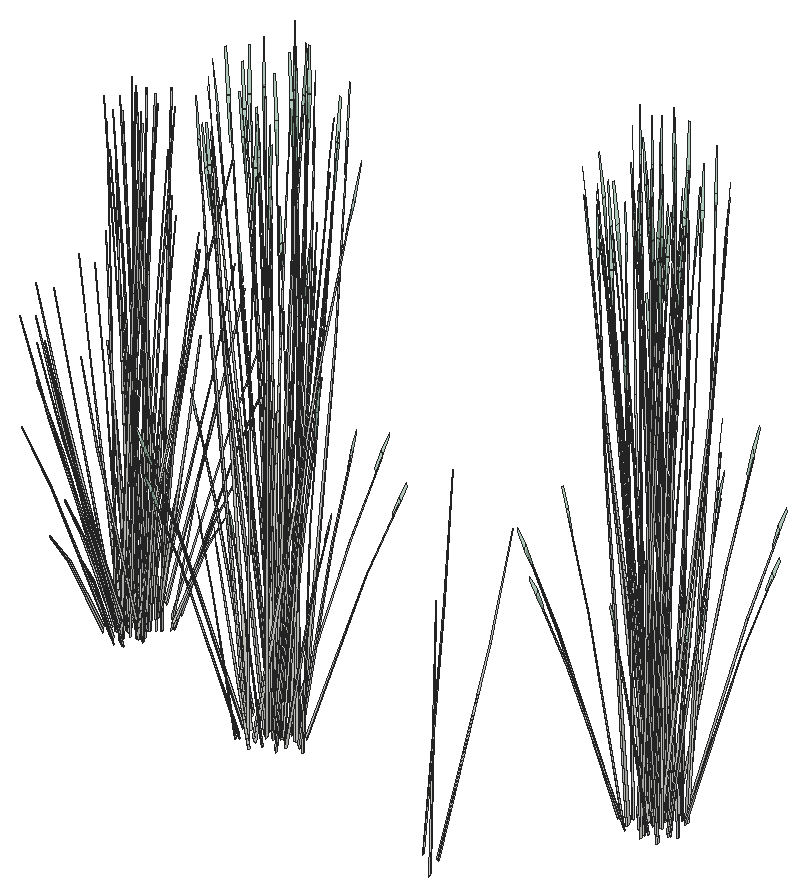
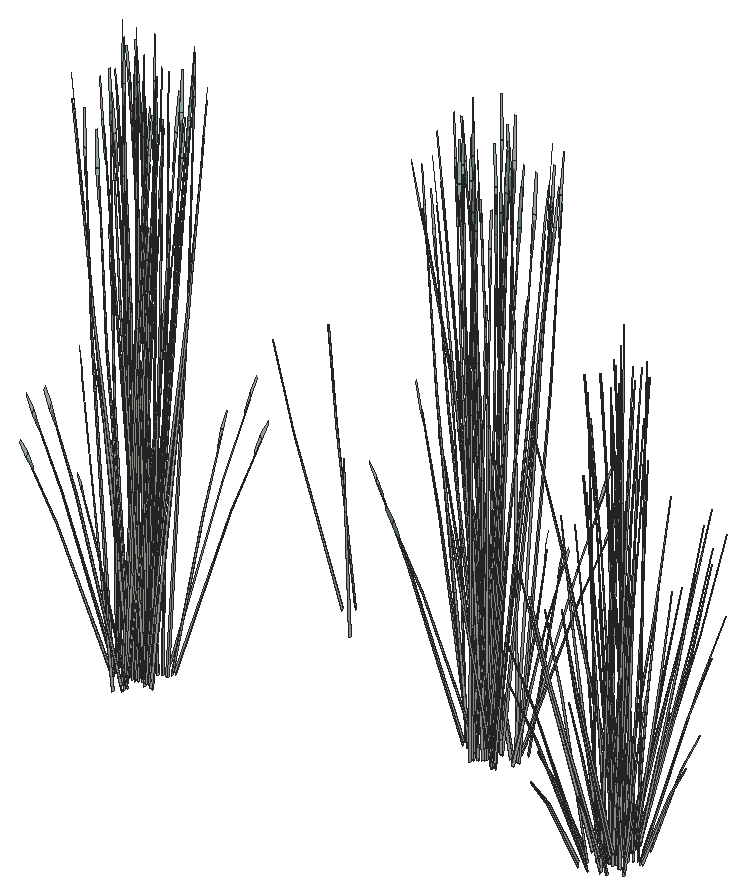
# SketchUp Ruby script. Lengths in inches.
U = 1.inch
M = Sketchup.active_model
def pt(a) = Geom::Point3d.new(a.map { |v| v * U })
def face(e, loops, mat)
  f = e.add_face(loops[0].map { |a| pt(a) })
  loops[1..].each { |l| e.add_face(l.map { |a| pt(a) }).erase! }
  f.material = f.back_material = mat if mat
  f
end
# faces: each face lists its corners as indices into pts; further lists are holes
def faces(e, pts, list, mat = nil) = list.each { |f| face(e, (f[0].is_a?(Array) ? f : [f]).map { |l| l.map { |i| pts[i] } }, mat) }
# xy, xz, yz: faces in a plane at the given z, y or x. An outline is a flat list of corners, or four numbers for a rectangle; further outlines are holes
def ring(l) = l.size == 4 ? [[l[0], l[1]], [l[2], l[1]], [l[2], l[3]], [l[0], l[3]]] : l.each_slice(2).to_a
def flat(e, list, mat, &to3) = list.each { |f| face(e, (f[0].is_a?(Array) ? f : [f]).map { |l| ring(l).map { |u, v| to3.(u, v) } }, mat) }
def xy(e, z, list, mat = nil) = flat(e, list, mat) { |x, y| [x, y, z] }
def xz(e, y, list, mat = nil) = flat(e, list, mat) { |x, z| [x, y, z] }
def yz(e, x, list, mat = nil) = flat(e, list, mat) { |y, z| [x, y, z] }
def lines(e, pts, list) = list.each { |a, b| e.add_line(pt(pts[a]), pt(pts[b])) }
# prism: a flat outline (further loops are holes) pulled along v
def prism(e, loops, v, mat = nil)
  f = face(e, loops, mat); d = Geom::Vector3d.new(v.map { |x| x * U })
  f.pushpull(f.normal.samedirection?(d) ? d.length : -d.length)
end
def box(e, o, s, mat = nil) = prism(e, [[o, [o[0] + s[0], o[1], o[2]], [o[0] + s[0], o[1] + s[1], o[2]], [o[0], o[1] + s[1], o[2]]]], [0, 0, s[2]], mat)
def at(x, y, z, deg = 0) = Geom::Transformation.translation(pt([x, y, z])) * Geom::Transformation.rotation(ORIGIN, Z_AXIS, deg.degrees)
def axes(o, x, y, z) = Geom::Transformation.new([*x, 0, *y, 0, *z, 0, *pt(o).to_a, 1])
def part(name) = M.definitions.add(name)
# library, detail: a bought-in or finely detailed component or shape, given as its bounding box
def library(name, o, s) = part(name).tap { |d| box(d.entities, o, s) }
def detail(e, o, s) = box(e.add_group.entities, o, s)
def put(e, d, t, mat = nil) = e.add_instance(d, t).tap { |i| i.material = mat if mat }
def group(e, t, mat = nil) = e.add_group.tap { |g| g.transformation = t; g.material = mat if mat }.entities
root = M.entities
M.materials.add("LightPink_Translucent").color = [175, 214, 192]
M.materials["LightPink_Translucent"].alpha = 0.75
c1 = part("blade")
p = [[2.15,0.21,22],[0,0.17,0],[0.09,0.45,0],[2.18,0.31,22],[2.29,0.31,22],[0.38,0.45,0],
  [2.48,0.24,33],[2.49,0.24,33],[2.48,0.22,33]]
faces(c1.entities,p,[[0,1,2,3],[4,5,2,3],[6,3,4,7],[8,0,3,6]])
c2 = part("blade with seeds\#1")
put(c2.entities,c1,at(0,0,0))
c3 = part("seeds")
p = [[0.3,-0.1,1.38],[-0.01,-0.03,1.59],[-0.01,-0.03,0.03],[0.14,-0.07,-0.07],[0.29,-0.03,3],[0.15,0.01,3.11]]
faces(c3.entities,p,[[0,1,2,3],[1,0,4,5]],"LightPink_Translucent")
c4 = part("blade with seeds")
put(c4.entities,c1,at(0,0,0))
put(c4.entities,c3,axes([2.4,0.25,30.99],[1.5799,-0.05474,1.17369],[-0.12525,1.92788,0.29478],[-0.07173,-0.02425,1.56792]))
put(root,c2,axes([484.83,550.86,141.1],[-0.01294,0.35246,-0.64693],[-0.54471,-0.02367,0.07807],[-0.05748,0.14932,0.91515]))
put(root,c2,axes([485.82,551.16,140.8],[0.23727,0.30983,-0.58282],[-0.48842,0.17267,0.07033],[0.05548,0.1497,0.82446]))
put(root,c2,axes([484.45,551.65,138.84],[0.15688,-0.06011,1.17311],[0.38733,0.18125,-0.25229],[-0.11528,0.15683,0.50157]))
put(root,c4,axes([464.21,558.03,139.62],[-0.13585,0.09014,1.30132],[-0.40687,-0.15777,-0.27986],[0.07542,-0.19621,0.55638]))
put(root,c4,axes([462.11,557.86,139.62],[-0.02894,0.14568,1.30132],[-0.4231,0.12195,-0.27986],[-0.0989,-0.1883,0.55638]))
put(root,c4,axes([462.46,558.39,139.42],[-0.29882,-0.44625,0],[0.49993,-0.24886,-0.46963],[0.11386,-0.05668,1.48977]))
put(root,c4,axes([463.11,557.85,139.2],[-0.33028,0.25548,-0.03542],[-0.30262,-0.27981,-0.16061],[-0.02131,-0.07928,0.52975]))
put(root,c4,axes([465.52,559.09,139.62],[-0.17074,-0.01319,1.30132],[-0.17492,-0.35385,-0.27986],[0.20976,-0.1001,0.55638]))
put(root,c4,axes([463.04,559.62,139.69],[-0.05569,-0.50815,-0.26477],[0.58006,-0.03072,-0.45502],[0.10214,-0.06769,1.45334]))
put(root,c4,axes([461.47,558.32,139.2],[-0.13787,0.36364,-0.03542],[-0.42434,-0.11186,-0.16061],[-0.06443,-0.05948,0.52975]))
put(root,c4,axes([462.78,560.15,139.69],[-0.53825,-0.21249,-0.26477],[0.25917,-0.44849,-0.45502],[-0.01692,-0.11011,1.45334]))
put(root,c4,axes([461.24,559.98,139.42],[-0.59763,0,0],[0,-0.49772,-0.46963],[0,-0.11336,1.48977]))
put(root,c4,axes([461.35,559.09,139.62],[0.09331,0.12399,1.30132],[-0.21502,0.33702,-0.27986],[-0.22079,-0.08055,0.55638]))
put(root,c4,axes([461.71,559.85,139.39],[-0.44456,0.37441,0.27988],[-0.44483,-0.37047,-0.33208],[-0.01552,-0.10632,1.50045]))
put(root,c4,axes([463.12,560.02,139.48],[0.53851,0.21584,0.21899],[-0.25917,0.44849,0.45502],[0,-0.10338,1.46094]))
put(root,c4,axes([462.91,560.625,139.48],[0.12668,-0.5277,-0.2132],[0.60063,0.09198,0.46656],[-0.10495,-0.07287,1.42361]))
put(root,c4,axes([464.66,558.5,139.43],[0.29882,-0.44625,0],[0.49993,0.24886,-0.46963],[0.11386,0.05668,1.48977]))
put(root,c4,axes([462.93,559.88,139.41],[0.2078,0.49797,0.41637],[-0.59373,0.17316,0.16339],[0.00726,-0.0915,1.44559]))
put(root,c4,axes([465.83,560.27,139.07],[-0.30783,0.05344,1.28841],[-0.049,-0.4254,0.07375],[0.2156,-0.06439,0.73315]))
put(root,c4,axes([466.39,559.89,139.32],[-0.29631,-0.28477,-0.05904],[0.32453,-0.26092,-0.26768],[0.09195,-0.01837,0.88292]))
put(root,c4,axes([463.68,559.93,139.27],[0,-0.51528,0],[0.59763,0,0],[0,0,1.63305]))
put(root,c4,axes([463.39,559.6,139.41],[-0.39628,0.40415,0.41637],[-0.4708,-0.35675,0.16339],[0.09554,-0.04033,1.44559]))
put(root,c4,axes([463.83,560.33,139.36],[-0.44456,-0.3833,-0.05579],[0.44483,-0.38354,0],[-0.01552,-0.01339,1.5977]))
put(root,c4,axes([462.5,559.29,138.72],[-0.47044,0.17829,1.17325],[-0.14973,-0.51157,0.45588],[0.28888,0.00851,1.33444]))
put(root,c4,axes([463.76,559.43,139.65],[0.0922,-0.39744,0.13176],[0.45047,0.06899,-0.37626],[0.08198,0.04081,1.15337]))
put(root,c4,axes([462.98,560.37,139.41],[0.60408,0.09383,0.41637],[-0.12294,0.52992,0.16339],[-0.08828,-0.05117,1.44559]))
put(root,c4,axes([463.71,559.56,139.69],[0.48255,-0.29566,-0.26477],[0.32089,0.41776,-0.45502],[0.11906,0.04243,1.45334]))
put(root,c4,axes([464.08,560.04,139.27],[0.53472,0,0],[0,0.46104,0],[0,0,1.6235]))
put(root,c4,axes([463.18,560.62,139.69],[-0.48255,0.29566,-0.26477],[-0.32089,-0.41776,-0.45502],[-0.11906,-0.04243,1.45334]))
put(root,c2,axes([446.29,564.22,138.9375],[-0.09372,0.11973,1.17311],[-0.31002,-0.15578,-0.25229],[0.042,-0.24224,0.50157]))
put(root,c4,axes([463.91,559.81,139.43],[-0.60408,-0.09383,0.44771],[0.12294,-0.52992,0.17569],[0.08828,0.05117,1.5544]))
put(root,c4,axes([463.43,561.12,139.27],[-0.15594,-0.38394,0],[0.4453,-0.13445,0],[0,0,1.40478]))
put(root,c4,axes([463.13,560.75,139.65],[-0.0922,0.39744,0.13176],[-0.45047,-0.06899,-0.37626],[-0.08198,-0.04081,1.15337]))
put(root,c4,axes([464.01,561.0625,139.25],[0.50177,-0.1511,-0.1747],[0.17632,0.43526,0.00007],[0.05539,-0.0167,1.58246]))
put(root,c4,axes([464.07,560.24,139.28],[0.33362,0.28765,0],[-0.33362,0.28765,0],[0,0,1.54032]))
put(root,c2,axes([445.78,564.89,140.9],[-0.16829,-0.43684,-0.58282],[0.34641,-0.24345,0.07033],[-0.03935,-0.21107,0.82446]))
put(root,c4,axes([463.32,561.29,139.26],[-0.48183,-0.19993,0],[0.23189,-0.41543,0],[0,0,1.48063]))
put(root,c4,axes([463.72,560.76,139.51],[-0.4667,-0.35844,-0.22925],[0.39271,-0.40249,0.50168],[-0.12567,0.04193,1.53076]))
put(root,c4,axes([492.18,564.85,139.53],[-0.03656,0.1661,1.30132],[-0.37341,0.10705,-0.27986],[-0.0699,-0.22562,0.55638]))
put(root,c4,axes([463.98,560.13,139.35],[0,0.51503,-0.0513],[-0.59763,0,0],[0,0.01619,1.63225]))
put(root,c2,axes([446.48,565.32,140.9],[0.00917,-0.49695,-0.58282],[0.38634,0.03338,0.07033],[0.04077,-0.21053,0.82446]))
put(root,c4,axes([462.23,561.68,139.42],[-0.29882,0.44625,0],[-0.49993,-0.24886,-0.46963],[-0.11386,-0.05668,1.48977]))
put(root,c2,axes([445.87,563.64,139.08],[0.06291,0.30716,0.94226],[-0.25998,-0.14458,0.69231],[0.01779,-0.16295,0.20754]))
put(root,c2,axes([444.74,564.64,138.9375],[-0.01129,0.1776,1.17311],[-0.30276,0.18194,-0.25229],[-0.08565,-0.21818,0.50157]))
put(root,c4,axes([464.27,559.99,139.65],[0.4453,-0.12987,0.13176],[0.15594,0.37086,-0.37626],[0,0.08162,1.15337]))
put(root,c2,axes([445.65,564.8,140.65],[-0.34661,-0.13468,-0.41919],[0.1188,-0.46175,-0.3247],[-0.03178,-0.18591,0.80208]))
put(root,c4,axes([465.92,560.9,139.62],[-0.1151,-0.10953,1.30132],[0.14976,-0.36232,-0.27986],[0.23288,0.04908,0.55638]))
put(root,c4,axes([493.98,565.49,139.53],[-0.12399,0.09331,1.30132],[-0.33702,-0.21502,-0.27986],[0.08055,-0.22079,0.55638]))
put(root,c4,axes([463.86,561.3,139.27],[0.48183,0.19993,0],[-0.23189,0.41543,0],[0,0,1.59208]))
put(root,c4,axes([464.06,561.74,139.26],[-0.29509,-0.44781,-0.04679],[0.49993,-0.24886,0.46963],[-0.12319,0.04264,1.48904]))
put(root,c4,axes([463.95,560.66,139.65],[0.3531,0.26757,0.13176],[-0.29453,0.30187,-0.37626],[-0.08198,0.04081,1.15337]))
put(root,c2,axes([445.02,565.01,140.9],[-0.30066,-0.25968,-0.58282],[0.21367,-0.45504,0.07033],[-0.10893,-0.15505,0.82446]))
put(root,c4,axes([463.69,561.13,139.35],[0.2078,0.51161,-0.05471],[-0.59373,0.17927,0],[0.00726,0.01787,1.56677]))
put(root,c4,axes([460.7,560.9,139.62],[0.1661,0.03656,1.30132],[0.10705,0.37341,-0.27986],[-0.22562,0.0699,0.55638]))
put(root,c4,axes([465.65,560.2,139.43],[0.59763,0,0],[0,0.49772,-0.46963],[0,0.11336,1.48977]))
put(root,c4,axes([465.41,560.46,139.27],[-0.59734,-0.00356,-0.04529],[0,-0.49772,0.45448],[-0.01877,0.1133,1.441]))
put(root,c4,axes([464.11,560.02,139.69],[0.53825,0.21249,-0.26477],[-0.25917,0.44849,-0.45502],[0.01692,0.11011,1.45334]))
put(root,c2,axes([444.1875,564.43,139.08],[0.19397,0.16559,0.94226],[-0.26061,0.14233,0.69231],[-0.0653,-0.13676,0.20754]))
put(root,c4,axes([463.84,560.56,139.69],[0.05569,0.50815,-0.26477],[-0.58006,0.03072,-0.45502],[-0.10214,0.06769,1.45334]))
put(root,c2,axes([444.88,565.03,140.65],[-0.34793,0.12771,-0.41919],[-0.06086,-0.48364,-0.3247],[-0.09345,-0.1386,0.80208]))
put(root,c4,axes([464.07,561.51,139.39],[0.59835,0.14475,0.27988],[-0.14969,0.51739,-0.33208],[-0.09903,0.06475,1.50045]))
put(root,c2,axes([446.92,565.98,140.65],[-0.09058,-0.49056,-0.41919],[0.34303,-0.08581,-0.3247],[0.0983,-0.13176,0.80208]))
put(root,c4,axes([464.43,561.79,139.42],[0.29882,0.44625,0],[-0.49993,0.24886,-0.46963],[-0.11386,0.05668,1.48977]))
put(root,c2,axes([447.27,565.3,139],[-0.01195,0.31879,0.86186],[-0.25381,-0.21053,0.47585],[0.09017,-0.12594,0.67605]))
put(root,c4,axes([491.39,566.375,139.33],[-0.44625,-0.29882,0],[0.24886,-0.49993,-0.46963],[0.05668,-0.11386,1.48977]))
put(root,c2,axes([446.77,565.35,139.08],[-0.10956,0.27991,0.94226],[-0.11132,-0.36143,0.69231],[0.0943,-0.09749,0.20754]))
put(root,c2,axes([446.66,566.35,138.9375],[-0.12631,-0.00877,1.17311],[-0.14109,-0.41923,-0.25229],[0.15118,-0.12942,0.50157]))
put(root,c4,axes([490.75,565.83,139.53],[0.07025,0.15082,1.30132],[-0.21183,0.37238,-0.27986],[-0.18329,-0.11083,0.55638]))
put(root,c4,axes([494.75,565.61,139.11],[-0.36364,-0.13787,-0.03542],[0.11186,-0.42434,-0.16061],[0.05948,-0.06443,0.52975]))
put(root,c4,axes([463.875,561.33,139.62],[0.00843,-0.14762,1.30132],[0.40305,-0.1649,-0.27986],[0.12442,0.17669,0.55638]))
put(root,c4,axes([495.21,566.25,139.53],[-0.14568,-0.02894,1.30132],[-0.12195,-0.4231,-0.27986],[0.1883,-0.0989,0.55638]))
put(root,c4,axes([492.45,567.32,139.6],[-0.29566,-0.48255,-0.26477],[0.41776,-0.32089,-0.45502],[0.04243,-0.11906,1.45334]))
put(root,c2,axes([444.41,565.65,140.9],[-0.35246,-0.01294,-0.58282],[0.02367,-0.54471,0.07033],[-0.14932,-0.05748,0.82446]))
put(root,c4,axes([493.09,565.39,139.33],[0,-0.59763,0],[0.49772,0,-0.46963],[0.11336,0,1.48977]))
put(root,c2,axes([444.4375,565.8,138.85],[-0.19052,0.46527,0.40731],[-0.34163,-0.2781,0],[0.04339,-0.10597,1.29208]))
put(root,c2,axes([445.63,564.88,138.85],[-0.38104,0,0.40731],[0,-0.5562,0],[0.08679,0,1.29208]))
put(root,c2,axes([445.03,566.47,138.96],[-0.34006,-0.0959,0.11878],[0.05903,-0.46856,-0.33919],[0.03492,-0.08527,1.03975]))
put(root,c4,axes([493.23,565.85,139.29],[-0.37441,-0.44456,0.27988],[0.37047,-0.44483,-0.33208],[0.10632,-0.01552,1.50045]))
put(root,c4,axes([461.79,561.99,139.83],[0.43418,-0.07886,0.05922],[0.09982,0.31771,-0.78537],[-0.02753,0.16083,0.70398]))
put(root,c4,axes([492.3125,567.86,139.41],[0.35844,-0.4667,-0.22925],[0.40249,0.39271,0.50168],[-0.04193,-0.12567,1.53076]))
put(root,c2,axes([443.83,566,138.9375],[0.07713,0.14131,1.17311],[-0.13499,0.4232,-0.25229],[-0.16789,-0.07845,0.50157]))
put(root,c2,axes([444.29,565.76,140.65],[-0.25603,0.35588,-0.41919],[-0.22422,-0.37594,-0.3247],[-0.13008,-0.05415,0.80208]))
put(root,c2,axes([445.12,566.67,139.04],[-0.31983,0.29864,0.36702],[-0.22522,-0.45236,-0.17663],[0.03957,-0.09664,1.17838]))
put(root,c2,axes([445.52,565.9375,138.96],[-0.11112,-0.46318,0.11878],[0.31732,-0.1622,-0.33919],[0.06984,0,1.03975]))
put(root,c4,axes([491.63,566.63,139.43],[-0.22267,0.44731,0.45182],[-0.39927,-0.26736,0],[0.05071,-0.10188,1.43328]))
put(root,c4,axes([492.44,567.05,139.39],[0.5277,0.12668,-0.2132],[-0.09198,0.60063,0.46656],[0.07287,-0.10495,1.42361]))
put(root,c2,axes([445.36,566.31,138.77],[-0.08028,0.62833,0.4036],[-0.45342,-0.12787,0.15838],[0.04378,-0.09182,1.40127]))
put(root,c4,axes([492.32,567.27,139.55],[-0.39744,-0.0922,0.13176],[0.06899,-0.45047,-0.37626],[0.04081,-0.08198,1.15337]))
put(root,c4,axes([461.6875,562.32,139.62],[0.15082,-0.07025,1.30132],[0.37238,0.21183,-0.27986],[-0.11083,0.18329,0.55638]))
put(root,c4,axes([493.02,565.75,139.43],[-0.44533,0,0.45182],[0,-0.53472,0],[0.10143,0,1.43328]))
put(root,c4,axes([491.33,568.2,139.17],[0.44781,-0.29509,-0.04679],[0.24886,0.49993,0.46963],[-0.04264,-0.12319,1.48904]))
put(root,c2,axes([445.4375,566.15,139.04],[-0.34335,-0.2412,0.36702],[0.16524,-0.50118,-0.17663],[0.07915,0,1.17838]))
put(root,c2,axes([447.08,567.07,140.65],[0.09552,-0.48869,-0.41919],[0.3275,0.16751,-0.3247],[0.13186,-0.04481,0.80208]))
put(root,c2,axes([445.73,566.14,138.63],[0.24613,-0.34702,0],[0.24613,0.34702,0],[0,0,1.38858]))
put(root,c2,axes([445.18,566.85,138.75],[0.3458,0.41219,0.37535],[-0.30525,0.4897,0.14729],[-0.03451,-0.09937,1.30318]))
put(root,c4,axes([492.92,566.92,139.6],[0.21249,-0.53825,-0.26477],[0.44849,0.25917,-0.45502],[0.11011,-0.01692,1.45334]))
put(root,c2,axes([444.63,565.97,138.84],[0.10113,0.5342,0.14473],[-0.37638,0.13191,0.28783],[0.05484,-0.04764,1.3159]))
put(root,c2,axes([443.22,566.52,139.08],[0.2222,-0.06377,0.94226],[-0.12306,0.35378,0.69231],[-0.11377,-0.03807,0.20754]))
put(root,c4,axes([491.09,565.93,139.74],[0.07886,0.43418,0.05922],[-0.31771,0.09982,-0.78537],[-0.16083,-0.02753,0.70398]))
put(root,c4,axes([492.51,567.99,139.6],[-0.50815,0.05569,-0.26477],[-0.03072,-0.58006,-0.45502],[-0.06769,-0.10214,1.45334]))
put(root,c2,axes([447.02,567.25,140.9],[0.30983,-0.23727,-0.58282],[0.17267,0.48842,0.07033],[0.1497,-0.05548,0.82446]))
put(root,c2,axes([445.62,565.2,138.84],[-0.27756,0.39059,0.14473],[-0.26921,-0.39362,0.28783],[0.05668,0.04314,1.3159]))
put(root,c4,axes([495.22,567.26,139.11],[-0.25548,-0.33028,-0.03542],[0.27981,-0.30262,-0.16061],[0.07928,-0.02131,0.52975]))
put(root,c4,axes([492.7,567.12,139.32],[-0.09383,0.60408,0.41637],[-0.52992,-0.12294,0.16339],[0.05117,-0.08828,1.44559]))
put(root,c2,axes([445.28,567.3125,139.04],[0.02352,0.53984,0.36702],[-0.39046,0.04882,-0.17663],[-0.03957,-0.09664,1.17838]))
put(root,c2,axes([444.61,567.5625,138.84],[0.37869,0.14361,0.14473],[-0.10717,0.52552,0.28783],[-0.00184,-0.09078,1.3159]))
put(root,c2,axes([445.54,567.13,138.81],[0.18468,-0.56014,0.19741],[0.38374,0.26958,0.41019],[-0.08846,0,1.31701]))
put(root,c4,axes([491.85,566.8,139.42],[0.1182,0.51358,0.16054],[-0.43988,0.12682,0.31929],[0.06409,-0.0458,1.4597]))
put(root,c4,axes([491.78,567.46,139.17],[0.19993,-0.48183,0],[0.41543,0.23189,0],[0,0,1.48063]))
put(root,c4,axes([491.28,568.57,139.33],[-0.44625,0.29882,0],[-0.24886,-0.49993,-0.46963],[-0.05668,-0.11386,1.48977]))
put(root,c2,axes([446.79,565.875,138.85],[-0.19052,-0.46527,0.40731],[0.34163,-0.2781,0],[0.04339,0.10597,1.29208]))
put(root,c4,axes([491.83,568.33,139.42],[0.44258,0.13807,0.16054],[-0.12525,0.50524,0.31929],[-0.00216,-0.08728,1.4597]))
put(root,c4,axes([492.42,568.09,139.55],[-0.26757,0.3531,0.13176],[-0.30187,-0.29453,-0.37626],[-0.04081,-0.08198,1.15337]))
put(root,c2,axes([445.42,567.33,138.75],[0.42608,-0.21614,0.37535],[0.14817,0.61757,0.14729],[-0.07829,-0.00755,1.30318]))
put(root,c4,axes([492.75,567.97,139.26],[0.3833,-0.44456,-0.05579],[0.38354,0.44483,0],[0.01339,-0.01552,1.5977]))
put(root,c2,axes([446.58,566.02,138.84],[-0.37869,-0.14361,0.14473],[0.10717,-0.52552,0.28783],[0.00184,0.09078,1.3159]))
put(root,c2,axes([445.91,566.28,139.04],[-0.02352,-0.53984,0.36702],[0.39046,-0.04882,-0.17663],[0.03957,0.09664,1.17838]))
put(root,c4,axes([491.5625,568.21,139.29],[-0.14475,0.59835,0.27988],[-0.51739,-0.14969,-0.33208],[-0.06475,-0.09903,1.50045]))
put(root,c2,axes([446.08,566.27,138.96],[0.22894,-0.36728,0.11878],[0.25829,0.30636,-0.33919],[0.03492,0.08527,1.03975]))
put(root,c4,axes([491.59,568.47,139.43],[0.22267,0.44731,0.45182],[-0.39927,0.26736,0],[-0.05071,-0.10188,1.43328]))
put(root,c4,axes([493.1875,567.07,139.32],[-0.49797,0.2078,0.41637],[-0.17316,-0.59373,0.16339],[0.0915,0.00726,1.44559]))
put(root,c4,axes([491.96,567.57,139.18],[0.38394,-0.15594,0],[0.13445,0.4453,0],[0,0,1.40478]))
put(root,c2,axes([446.5625,567.61,138.84],[-0.10113,-0.5342,0.14473],[0.37638,-0.13191,0.28783],[-0.05484,0.04764,1.3159]))
put(root,c2,axes([444.1,566.64,140.9],[-0.30983,0.23727,-0.58282],[-0.17267,-0.48842,0.07033],[-0.1497,0.05548,0.82446]))
put(root,c2,axes([445.76,567.4375,139.04],[0.34335,0.2412,0.36702],[-0.16524,0.50118,-0.17663],[-0.07915,0,1.17838]))
put(root,c4,axes([492.96,569.12,139.42],[0.32439,-0.37551,0.16054],[0.31463,0.37842,0.31929],[-0.06625,-0.04147,1.4597]))
put(root,c4,axes([493.14,567.82,139.18],[0.51528,0,0],[0,0.59763,0],[0,0,1.63305]))
put(root,c4,axes([493.05,567.26,139.38],[-0.21584,0.53851,0.21899],[-0.44849,-0.25917,0.45502],[0.10338,0,1.46094]))
put(root,c4,axes([492.9375,568.12,139.26],[-0.51503,0,-0.0513],[0,-0.59763,0],[-0.01619,0,1.63225]))
put(root,c2,axes([445.84,567.28,138.75],[0.08028,-0.62833,0.37535],[0.45342,0.12787,0.14729],[-0.04378,0.09182,1.30318]))
put(root,c2,axes([444.04,566.82,140.65],[-0.09552,0.48869,-0.41919],[-0.3275,-0.16751,-0.3247],[-0.13186,0.04481,0.80208]))
put(root,c4,axes([494.13,566.85,139.42],[-0.44258,-0.13807,0.16054],[0.12525,-0.50524,0.31929],[0.00216,0.08728,1.4597]))
put(root,c4,axes([491.94,567.83,139.25],[-0.51161,0.2078,-0.05471],[-0.17927,-0.59373,0],[-0.01787,0.00726,1.56677]))
put(root,c2,axes([445.54,566.03,139.14],[-0.35877,0.01358,1.15892],[0.093,-0.61462,0.4907],[0.19631,0.14537,1.09393]))
put(root,c4,axes([494.68,566.6,139.33],[0.44625,-0.29882,0],[0.24886,0.49993,-0.46963],[0.05668,0.11386,1.48977]))
put(root,c4,axes([492.61,569.55,139.17],[0.00356,-0.59734,-0.04529],[0.49772,0,0.45448],[-0.1133,-0.01877,1.441]))
put(root,c2,axes([447.22,568.51,139.13],[-0.06748,-0.45162,0.05338],[0.27185,-0.10383,-0.708],[0.13761,0.02863,0.63462]))
put(root,c4,axes([494.11,568.375,139.42],[-0.1182,-0.51358,0.16054],[0.43988,-0.12682,0.31929],[-0.06409,0.0458,1.4597]))
put(root,c4,axes([493.47,567.53,139.32],[-0.40415,-0.39628,0.41637],[0.35675,-0.4708,0.16339],[0.04033,0.09554,1.44559]))
put(root,c4,axes([492.83,568.21,139.19],[-0.28765,0.33362,0],[-0.28765,-0.33362,0],[0,0,1.54032]))
put(root,c4,axes([491.77,568.01,139.18],[-0.19993,0.48183,0],[-0.41543,-0.23189,0],[0,0,1.59208]))
put(root,c2,axes([446.16,567.12,138.96],[0.34006,0.0959,0.11878],[-0.05903,0.46856,-0.33919],[-0.03492,0.08527,1.03975]))
put(root,c4,axes([493.26,568.05,139.34],[0.09383,-0.60408,0.44771],[0.52992,0.12294,0.17569],[-0.05117,0.08828,1.5544]))
put(root,c2,axes([445.57,568.7,138.85],[0.38104,0,0.40731],[0,0.5562,0],[-0.08679,0,1.29208]))
put(root,c4,axes([493.03,568.22,139.18],[0,0.53472,0],[-0.46104,0,0],[0,0,1.6235]))
put(root,c2,axes([446.76,567.79,138.85],[0.19052,-0.46527,0.40731],[0.34163,0.2781,0],[-0.04339,0.10597,1.29208]))
put(root,c4,axes([493.45,567.1875,139.6],[0.50815,-0.05569,-0.26477],[0.03072,0.58006,-0.45502],[0.06769,0.10214,1.45334]))
put(root,c4,axes([493.08,568.41,139.55],[0.12987,0.4453,0.13176],[-0.37086,0.15594,-0.37626],[-0.08162,0,1.15337]))
put(root,c2,axes([447.71,568.25,139.08],[-0.22657,0.01287,0.94226],[0.1616,-0.32149,0.69231],[0.10799,0.06323,0.20754]))
put(root,c4,axes([493.05,568.26,139.6],[-0.21249,0.53825,-0.26477],[-0.44849,-0.25917,-0.45502],[-0.11011,0.01692,1.45334]))
put(root,c4,axes([495.04,568.35,139.53],[-0.09014,-0.13585,1.30132],[0.15777,-0.40687,-0.27986],[0.19621,0.07542,0.55638]))
put(root,c2,axes([443.49,568.34,139.08],[0.13262,-0.25932,0.94226],[0.07972,0.37767,0.69231],[-0.10192,0.08081,0.20754]))
put(root,c4,axes([492.94,569.42,139.43],[0.44533,0,0.45182],[0,0.53472,0],[-0.10143,0,1.43328]))
put(root,c4,axes([493.64,567.9,139.55],[0.39744,0.0922,0.13176],[-0.06899,0.45047,-0.37626],[-0.04081,0.08198,1.15337]))
put(root,c4,axes([494.34,568.54,139.43],[0.22267,-0.44731,0.45182],[0.39927,0.26736,0],[-0.05071,0.10188,1.43328]))
put(root,c4,axes([492.01,568.15,139.16],[0.1511,0.50177,-0.1747],[-0.43526,0.17632,0.00007],[0.0167,0.05539,1.58246]))
put(root,c2,axes([443.6875,568.1875,138.9375],[0.12465,0.0301,1.17311],[0.10435,0.44009,-0.25229],[-0.16111,0.10287,0.50157]))
put(root,c2,axes([447.51,568.62,138.9375],[-0.06011,-0.15688,1.17311],[0.18125,-0.38733,-0.25229],[0.15683,0.11528,0.50157]))
put(root,c4,axes([491.74,568.02,139.53],[0.14762,0.00843,1.30132],[0.1649,0.40305,-0.27986],[-0.17669,0.12442,0.55638]))
put(root,c4,axes([492.87,569.79,139.33],[0,0.59763,0],[-0.49772,0,-0.46963],[-0.11336,0,1.48977]))
put(root,c2,axes([444.19,567.71,140.9],[-0.18418,0.4239,-0.58282],[-0.32274,-0.30126,0.07033],[-0.10997,0.15358,0.82446]))
put(root,c2,axes([444.2,567.91,140.65],[0.09058,0.49056,-0.41919],[-0.34303,0.08581,-0.3247],[-0.0983,0.13176,0.80208]))
put(root,c4,axes([493.51,567.86,139.6],[0.29566,0.48255,-0.26477],[-0.41776,0.32089,-0.45502],[-0.04243,0.11906,1.45334]))
put(root,c2,axes([446.25,568.87,140.65],[0.34793,-0.12771,-0.41919],[0.06086,0.48364,-0.3247],[0.09345,0.1386,0.80208]))
put(root,c4,axes([494.57,568.8,139.33],[0.44625,0.29882,0],[-0.24886,0.49993,-0.46963],[-0.05668,0.11386,1.48977]))
put(root,c2,axes([445.06,569.55,139.08],[-0.02727,-0.31739,0.94226],[0.24024,0.20133,0.69231],[-0.03604,0.15684,0.20754]))
put(root,c4,axes([493.18,570.54,139.23],[0.28477,-0.29631,-0.05904],[0.26092,0.32453,-0.26768],[0.01837,0.09195,0.88292]))
put(root,c2,axes([446.96,570,139.08],[-0.1727,-0.20718,0.94226],[0.27339,-0.08175,0.69231],[0.04895,0.14972,0.20754]))
put(root,c2,axes([444.72,568.74,140.65],[0.25241,0.36098,-0.41919],[-0.26664,0.31614,-0.3247],[-0.0384,0.18341,0.80208]))
put(root,c2,axes([445.47,569.09,140.65],[0.34661,0.13468,-0.41919],[-0.1188,0.46175,-0.3247],[0.03178,0.18591,0.80208]))
put(root,c2,axes([444.65,568.58,140.9],[-0.00917,0.49695,-0.58282],[-0.38634,-0.03338,0.07033],[-0.04077,0.21053,0.82446]))
put(root,c2,axes([444.74,568.98,138.9375],[0.10609,-0.09706,1.17311],[0.28837,0.22366,-0.25229],[-0.06892,0.22965,0.50157]))
put(root,c4,axes([493.98,569.66,139.53],[0.01319,-0.17074,1.30132],[0.35385,-0.17492,-0.27986],[0.1001,0.20976,0.55638]))
put(root,c2,axes([446.29,569.64,138.9375],[0.03128,-0.17277,1.17311],[0.3195,-0.11135,-0.25229],[0.05981,0.23468,0.50157]))
put(root,c4,axes([492.8,569.98,138.97],[-0.05344,-0.30783,1.28841],[0.4254,-0.049,0.07375],[0.06439,0.2156,0.73315]))
put(root,c4,axes([492.17,570.0625,139.53],[0.10953,-0.1151,1.30132],[0.36232,0.14976,-0.27986],[-0.04908,0.23288,0.55638]))
